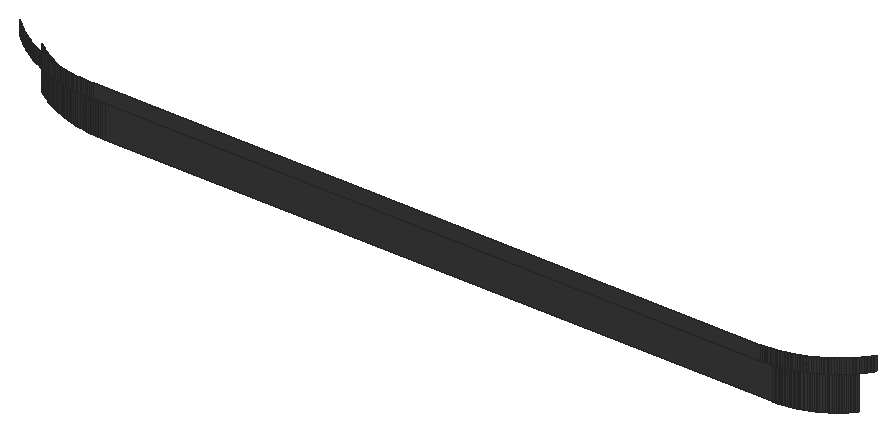
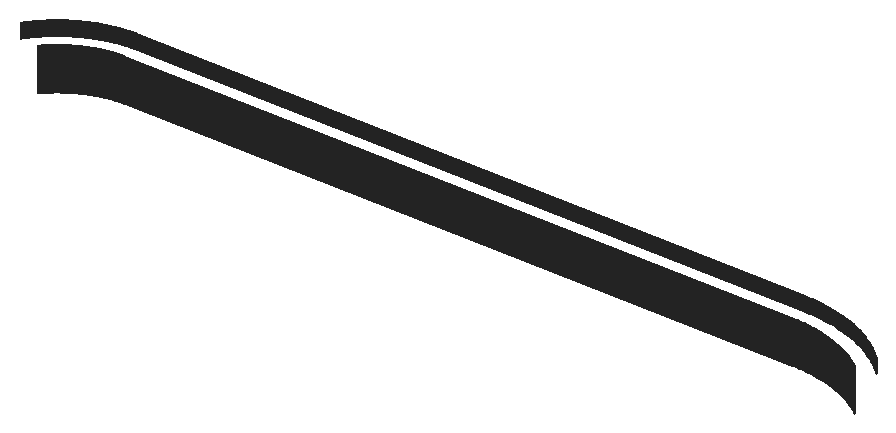
# SketchUp Ruby script. Lengths in inches.
U = 1.inch
M = Sketchup.active_model
def pt(a) = Geom::Point3d.new(a.map { |v| v * U })
def face(e, loops, mat)
  f = e.add_face(loops[0].map { |a| pt(a) })
  loops[1..].each { |l| e.add_face(l.map { |a| pt(a) }).erase! }
  f.material = f.back_material = mat if mat
  f
end
# faces: each face lists its corners as indices into pts; further lists are holes
def faces(e, pts, list, mat = nil) = list.each { |f| face(e, (f[0].is_a?(Array) ? f : [f]).map { |l| l.map { |i| pts[i] } }, mat) }
# xy, xz, yz: faces in a plane at the given z, y or x. An outline is a flat list of corners, or four numbers for a rectangle; further outlines are holes
def ring(l) = l.size == 4 ? [[l[0], l[1]], [l[2], l[1]], [l[2], l[3]], [l[0], l[3]]] : l.each_slice(2).to_a
def flat(e, list, mat, &to3) = list.each { |f| face(e, (f[0].is_a?(Array) ? f : [f]).map { |l| ring(l).map { |u, v| to3.(u, v) } }, mat) }
def xy(e, z, list, mat = nil) = flat(e, list, mat) { |x, y| [x, y, z] }
def xz(e, y, list, mat = nil) = flat(e, list, mat) { |x, z| [x, y, z] }
def yz(e, x, list, mat = nil) = flat(e, list, mat) { |y, z| [x, y, z] }
def lines(e, pts, list) = list.each { |a, b| e.add_line(pt(pts[a]), pt(pts[b])) }
# prism: a flat outline (further loops are holes) pulled along v
def prism(e, loops, v, mat = nil)
  f = face(e, loops, mat); d = Geom::Vector3d.new(v.map { |x| x * U })
  f.pushpull(f.normal.samedirection?(d) ? d.length : -d.length)
end
def box(e, o, s, mat = nil) = prism(e, [[o, [o[0] + s[0], o[1], o[2]], [o[0] + s[0], o[1] + s[1], o[2]], [o[0], o[1] + s[1], o[2]]]], [0, 0, s[2]], mat)
def at(x, y, z, deg = 0) = Geom::Transformation.translation(pt([x, y, z])) * Geom::Transformation.rotation(ORIGIN, Z_AXIS, deg.degrees)
def axes(o, x, y, z) = Geom::Transformation.new([*x, 0, *y, 0, *z, 0, *pt(o).to_a, 1])
def part(name) = M.definitions.add(name)
# library, detail: a bought-in or finely detailed component or shape, given as its bounding box
def library(name, o, s) = part(name).tap { |d| box(d.entities, o, s) }
def detail(e, o, s) = box(e.add_group.entities, o, s)
def put(e, d, t, mat = nil) = e.add_instance(d, t).tap { |i| i.material = mat if mat }
def group(e, t, mat = nil) = e.add_group.tap { |g| g.transformation = t; g.material = mat if mat }.entities
root = M.entities
M.materials.add("1496 AP 8293 CARBON COPY").color = [58, 58, 58]
xz(root,64,[[43.57,270,44,273],[44,270,185,273],[185,270,185.27,273]],"1496 AP 8293 CARBON COPY")
xz(root,67,[[43.61,261,44,270],[44,261,185,270],[185,261,185.24,270]],"1496 AP 8293 CARBON COPY")
xz(root,67.01,[[185.47,261,185.71,270]],"1496 AP 8293 CARBON COPY")
p = [[42.43,67.04,261],[42.43,67.04,270],[42.04,67.0625,270],[42.04,67.0625,261],[42.82,67.02,261],[42.82,67.02,270],
  [43.21,67.01,261],[43.21,67.01,270],[43.61,67,261],[43.61,67,270],[185.47,67.01,261],[185.47,67.01,270],
  [185.24,67,270],[185.24,67,261],[185.94,67.02,261],[185.94,67.02,270],[185.71,67.01,270],[185.71,67.01,261],
  [186.18,67.04,261],[186.18,67.04,270],[186.41,67.06,261],[186.41,67.06,270],[41.25,67.125,261],[41.25,67.125,270],
  [40.86,67.16,270],[40.86,67.16,261],[41.65,67.09,261],[41.65,67.09,270],[186.65,67.08,261],[186.65,67.08,270],
  [186.88,67.1,261],[186.88,67.1,270],[187.12,67.125,261],[187.12,67.125,270],[187.35,67.15,261],[187.35,67.15,270],
  [40.47,67.21,261],[40.47,67.21,270],[40.08,67.26,270],[40.08,67.26,261],[187.58,67.1875,261],[187.58,67.1875,270],
  [187.82,67.22,261],[187.82,67.22,270],[188.05,67.26,261],[188.05,67.26,270],[39.7,67.31,261],[39.7,67.31,270],
  [39.31,67.37,270],[39.31,67.37,261],[188.28,67.3,261],[188.28,67.3,270],[188.51,67.35,261],[188.51,67.35,270],
  [188.74,67.39,261],[188.74,67.39,270],[38.92,67.43,261],[38.92,67.43,270],[38.53,67.5,270],[38.53,67.5,261],
  [188.97,67.44,261],[188.97,67.44,270],[189.2,67.5,261],[189.2,67.5,270],[38.15,67.58,270],[38.15,67.58,261],
  [189.43,67.55,261],[189.43,67.55,270],[37.76,67.66,270],[37.76,67.66,261],[189.66,67.61,261],[189.66,67.61,270],
  [189.89,67.68,261],[189.89,67.68,270],[37.38,67.74,261],[37.38,67.74,270],[37,67.83,270],[37,67.83,261],
  [190.11,67.74,261],[190.11,67.74,270],[190.34,67.81,261],[190.34,67.81,270],[36.62,67.92,270],[36.62,67.92,261],
  [190.5625,67.88,261],[190.5625,67.88,270],[36.24,68.02,270],[36.24,68.02,261],[190.79,67.96,261],[190.79,67.96,270],
  [35.86,68.125,270],[35.86,68.125,261],[191.01,68.03,261],[191.01,68.03,270],[191.23,68.11,261],[191.23,68.11,270],
  [35.48,68.24,270],[35.48,68.24,261],[191.45,68.2,261],[191.45,68.2,270],[35.1,68.35,270],[35.1,68.35,261],
  [191.67,68.28,261],[191.67,68.28,270],[34.73,68.47,270],[34.73,68.47,261],[191.89,68.37,261],[191.89,68.37,270],
  [192.11,68.46,261],[192.11,68.46,270],[34.36,68.59,270],[34.36,68.59,261],[192.32,68.56,261],[192.32,68.56,270],
  [33.99,68.72,270],[33.99,68.72,261],[192.54,68.65,261],[192.54,68.65,270],[33.62,68.85,270],[33.62,68.85,261],
  [192.75,68.75,261],[192.75,68.75,270],[192.96,68.86,261],[192.96,68.86,270],[33.25,68.99,270],[33.25,68.99,261],
  [193.17,68.96,261],[193.17,68.96,270],[32.88,69.14,270],[32.88,69.14,261],[193.38,69.07,261],[193.38,69.07,270],
  [32.52,69.28,270],[32.52,69.28,261],[193.59,69.18,261],[193.59,69.18,270],[193.8,69.3,261],[193.8,69.3,270],
  [32.16,69.4375,270],[32.16,69.4375,261],[194,69.41,261],[194,69.41,270],[31.8,69.59,270],[31.8,69.59,261],
  [194.2,69.53,261],[194.2,69.53,270],[194.4,69.65,261],[194.4,69.65,270],[31.44,69.76,270],[31.44,69.76,261],
  [194.61,69.78,261],[194.61,69.78,270],[31.08,69.92,270],[31.08,69.92,261],[194.8,69.9,261],[194.8,69.9,270],
  [30.73,70.09,270],[30.73,70.09,261],[195,70.03,261],[195,70.03,270],[195.2,70.17,261],[195.2,70.17,270],
  [30.38,70.27,270],[30.38,70.27,261],[195.39,70.3,261],[195.39,70.3,270],[30.03,70.45,270],[30.03,70.45,261],
  [195.58,70.4375,261],[195.58,70.4375,270],[195.77,70.58,261],[195.77,70.58,270],[29.69,70.64,270],[29.69,70.64,261],
  [29.34,70.83,270],[29.34,70.83,261],[195.96,70.72,261],[195.96,70.72,270],[196.14,70.86,261],[196.14,70.86,270],
  [29,71.02,270],[29,71.02,261],[196.33,71.01,261],[196.33,71.01,270],[28.66,71.22,270],[28.66,71.22,261],
  [196.51,71.16,261],[196.51,71.16,270],[28.33,71.42,270],[28.33,71.42,261],[196.69,71.3125,261],[196.69,71.3125,270],
  [196.87,71.47,261],[196.87,71.47,270],[27.99,71.63,270],[27.99,71.63,261],[197.04,71.625,261],[197.04,71.625,270],
  [27.66,71.84,270],[27.66,71.84,261],[197.22,71.78,261],[197.22,71.78,270],[27.33,72.06,270],[27.33,72.06,261],
  [197.39,71.94,261],[197.39,71.94,270],[197.56,72.11,261],[197.56,72.11,270],[27.01,72.28,270],[27.01,72.28,261],
  [197.73,72.27,261],[197.73,72.27,270],[26.6875,72.5,270],[26.6875,72.5,261],[197.89,72.44,261],[197.89,72.44,270],
  [198.06,72.61,261],[198.06,72.61,270],[26.37,72.73,270],[26.37,72.73,261],[198.22,72.78,261],[198.22,72.78,270],
  [26.05,72.96,270],[26.05,72.96,261],[198.375,72.96,261],[198.375,72.96,270],[25.74,73.2,270],[25.74,73.2,261],
  [198.53,73.13,261],[198.53,73.13,270],[41.84,64.07,270],[42.27,64.05,270],[42.27,64.05,273],[41.84,64.07,273],
  [42.7,64.03,270],[42.7,64.03,273],[43.14,64.01,270],[43.14,64.01,273],[43.57,64,270],[43.57,64,273],
  [185.27,64,270],[185.55,64.01,270],[185.55,64.01,273],[185.27,64,273],[185.82,64.02,270],[185.82,64.02,273],
  [186.1,64.03,270],[186.1,64.03,273],[186.375,64.04,270],[186.375,64.04,273],[186.65,64.06,270],[186.65,64.06,273],
  [40.55,64.18,270],[40.98,64.14,270],[40.98,64.14,273],[40.55,64.18,273],[41.41,64.1,270],[41.41,64.1,273],
  [186.92,64.09,270],[186.92,64.09,273],[187.2,64.12,270],[187.2,64.12,273],[187.47,64.15,270],[187.47,64.15,273],
  [187.74,64.18,270],[187.74,64.18,273],[39.69,64.28,270],[40.12,64.23,270],[40.12,64.23,273],[39.69,64.28,273],
  [188.01,64.22,270],[188.01,64.22,273],[188.29,64.26,270],[188.29,64.26,273],[38.84,64.41,270],[39.26,64.34,270],
  [39.26,64.34,273],[38.84,64.41,273],[188.56,64.3,270],[188.56,64.3,273],[188.83,64.35,270],[188.83,64.35,273],
  [38.41,64.48,270],[38.41,64.48,273],[189.1,64.4,270],[189.1,64.4,273],[189.37,64.46,270],[189.37,64.46,273],
  [37.99,64.55,270],[37.99,64.55,273],[189.63,64.52,270],[189.63,64.52,273],[189.9,64.58,270],[189.9,64.58,273],
  [37.14,64.72,270],[37.5625,64.63,270],[37.5625,64.63,273],[37.14,64.72,273],[190.17,64.65,270],[190.17,64.65,273],
  [190.44,64.72,270],[190.44,64.72,273],[36.72,64.8125,270],[36.72,64.8125,273],[190.7,64.79,270],[190.7,64.79,273],
  [36.3,64.91,270],[36.3,64.91,273],[190.96,64.86,270],[190.96,64.86,273],[35.875,65.02,270],[35.875,65.02,273],
  [191.23,64.94,270],[191.23,64.94,273],[191.49,65.03,270],[191.49,65.03,273],[35.46,65.125,270],[35.46,65.125,273],
  [191.75,65.11,270],[191.75,65.11,273],[35.04,65.24,270],[35.04,65.24,273],[192.01,65.2,270],[192.01,65.2,273],
  [34.63,65.36,270],[34.63,65.36,273],[192.27,65.3,270],[192.27,65.3,273],[192.53,65.39,270],[192.53,65.39,273],
  [34.21,65.48,270],[34.21,65.48,273],[192.78,65.49,270],[192.78,65.49,273],[33.8,65.62,270],[33.8,65.62,273],
  [193.04,65.6,270],[193.04,65.6,273],[33.39,65.75,270],[33.39,65.75,273],[193.29,65.71,270],[193.29,65.71,273],
  [193.54,65.82,270],[193.54,65.82,273],[32.98,65.89,270],[32.98,65.89,273],[193.79,65.93,270],[193.79,65.93,273],
  [32.58,66.04,270],[32.58,66.04,273],[194.04,66.05,270],[194.04,66.05,273],[32.17,66.19,270],[32.17,66.19,273],
  [194.29,66.17,270],[194.29,66.17,273],[31.77,66.35,270],[31.77,66.35,273],[194.53,66.29,270],[194.53,66.29,273],
  [31.37,66.51,270],[31.37,66.51,273],[194.78,66.42,270],[194.78,66.42,273],[195.02,66.54,270],[195.02,66.54,273],
  [30.97,66.68,270],[30.97,66.68,273],[195.26,66.68,270],[195.26,66.68,273],[30.58,66.85,270],[30.58,66.85,273],
  [195.5,66.8125,270],[195.5,66.8125,273],[195.74,66.95,270],[195.74,66.95,273],[30.18,67.03,270],[30.18,67.03,273],
  [29.79,67.21,270],[29.79,67.21,273],[195.97,67.09,270],[195.97,67.09,273],[196.21,67.24,270],[196.21,67.24,273],
  [29.4,67.4,270],[29.4,67.4,273],[196.4375,67.39,270],[196.4375,67.39,273],[29.02,67.6,270],[29.02,67.6,273],
  [196.67,67.54,270],[196.67,67.54,273],[196.89,67.69,270],[196.89,67.69,273],[28.63,67.8,270],[28.63,67.8,273],
  [197.12,67.85,270],[197.12,67.85,273],[28.25,68,270],[28.25,68,273],[197.34,68.01,270],[197.34,68.01,273],
  [27.875,68.21,270],[27.875,68.21,273],[197.56,68.17,270],[197.56,68.17,273],[27.5,68.42,270],[27.5,68.42,273],
  [197.78,68.34,270],[197.78,68.34,273],[198,68.51,270],[198,68.51,273],[27.13,68.64,270],[27.13,68.64,273],
  [198.22,68.68,270],[198.22,68.68,273],[26.76,68.86,270],[26.76,68.86,273],[198.43,68.85,270],[198.43,68.85,273],
  [26.39,69.09,270],[26.39,69.09,273],[198.64,69.03,270],[198.64,69.03,273],[198.85,69.21,270],[198.85,69.21,273],
  [26.03,69.32,270],[26.03,69.32,273],[199.05,69.39,270],[199.05,69.39,273],[25.67,69.5625,270],[25.67,69.5625,273],
  [199.25,69.58,270],[199.25,69.58,273],[25.31,69.8,270],[25.31,69.8,273],[199.46,69.77,270],[199.46,69.77,273],
  [24.95,70.05,270],[24.95,70.05,273],[199.65,69.96,270],[199.65,69.96,273],[199.85,70.15,270],[199.85,70.15,273],
  [24.6,70.3,270],[24.6,70.3,273],[200.04,70.35,270],[200.04,70.35,273],[24.26,70.56,270],[24.26,70.56,273],
  [200.23,70.54,270],[200.23,70.54,273],[200.42,70.75,270],[200.42,70.75,273],[23.91,70.82,270],[23.91,70.82,273],
  [200.61,70.95,270],[200.61,70.95,273],[23.57,71.08,270],[23.57,71.08,273],[200.79,71.15,270],[200.79,71.15,273],
  [23.23,71.35,270],[23.23,71.35,273],[200.97,71.36,270],[200.97,71.36,273],[22.9,71.63,270],[22.9,71.63,273],
  [201.15,71.57,270],[201.15,71.57,273],[22.57,71.91,270],[22.57,71.91,273],[201.32,71.78,270],[201.32,71.78,273],
  [201.49,72,270],[201.49,72,273],[22.24,72.1875,270],[22.24,72.1875,273],[201.66,72.22,270],[201.66,72.22,273],
  [21.92,72.48,270],[21.92,72.48,273],[201.83,72.44,270],[201.83,72.44,273],[201.99,72.66,270],[201.99,72.66,273],
  [21.6,72.77,270],[21.6,72.77,273],[202.15,72.88,270],[202.15,72.88,273],[21.28,73.0625,270],[21.28,73.0625,273],
  [202.31,73.11,270],[202.31,73.11,273]]
faces(root,p,[[0,1,2,3],[4,5,1,0],[6,7,5,4],[8,9,7,6],[10,11,12,13],[14,15,16,17],[18,19,15,14],[20,21,19,18],
  [22,23,24,25],[26,27,23,22],[3,2,27,26],[28,29,21,20],[30,31,29,28],[32,33,31,30],[34,35,33,32],[36,37,38,39],
  [25,24,37,36],[40,41,35,34],[42,43,41,40],[44,45,43,42],[46,47,48,49],[39,38,47,46],[50,51,45,44],[52,53,51,50],
  [54,55,53,52],[56,57,58,59],[49,48,57,56],[60,61,55,54],[62,63,61,60],[59,58,64,65],[66,67,63,62],[65,64,68,69],
  [70,71,67,66],[72,73,71,70],[74,75,76,77],[69,68,75,74],[78,79,73,72],[80,81,79,78],[77,76,82,83],[84,85,81,80],
  [83,82,86,87],[88,89,85,84],[87,86,90,91],[92,93,89,88],[94,95,93,92],[91,90,96,97],[98,99,95,94],[97,96,100,101],
  [102,103,99,98],[101,100,104,105],[106,107,103,102],[108,109,107,106],[105,104,110,111],[112,113,109,108],[111,110,114,115],[116,117,113,112],
  [115,114,118,119],[120,121,117,116],[122,123,121,120],[119,118,124,125],[126,127,123,122],[125,124,128,129],[130,131,127,126],[129,128,132,133],
  [134,135,131,130],[136,137,135,134],[133,132,138,139],[140,141,137,136],[139,138,142,143],[144,145,141,140],[146,147,145,144],[143,142,148,149],
  [150,151,147,146],[149,148,152,153],[154,155,151,150],[153,152,156,157],[158,159,155,154],[160,161,159,158],[157,156,162,163],[164,165,161,160],
  [163,162,166,167],[168,169,165,164],[170,171,169,168],[167,166,172,173],[173,172,174,175],[176,177,171,170],[178,179,177,176],[175,174,180,181],
  [182,183,179,178],[181,180,184,185],[186,187,183,182],[185,184,188,189],[190,191,187,186],[192,193,191,190],[189,188,194,195],[196,197,193,192],
  [195,194,198,199],[200,201,197,196],[199,198,202,203],[204,205,201,200],[206,207,205,204],[203,202,208,209],[210,211,207,206],[209,208,212,213],
  [214,215,211,210],[216,217,215,214],[213,212,218,219],[220,221,217,216],[219,218,222,223],[224,225,221,220],[223,222,226,227],[228,229,225,224],
  [230,231,232,233],[231,234,235,232],[234,236,237,235],[236,238,239,237],[240,241,242,243],[241,244,245,242],[244,246,247,245],[246,248,249,247],
  [248,250,251,249],[252,253,254,255],[253,256,257,254],[256,230,233,257],[250,258,259,251],[258,260,261,259],[260,262,263,261],[262,264,265,263],
  [266,267,268,269],[267,252,255,268],[264,270,271,265],[270,272,273,271],[274,275,276,277],[275,266,269,276],[272,278,279,273],[278,280,281,279],
  [282,274,277,283],[280,284,285,281],[284,286,287,285],[288,282,283,289],[286,290,291,287],[290,292,293,291],[294,295,296,297],[295,288,289,296],
  [292,298,299,293],[298,300,301,299],[302,294,297,303],[300,304,305,301],[306,302,303,307],[304,308,309,305],[310,306,307,311],[308,312,313,309],
  [312,314,315,313],[316,310,311,317],[314,318,319,315],[320,316,317,321],[318,322,323,319],[324,320,321,325],[322,326,327,323],[326,328,329,327],
  [330,324,325,331],[328,332,333,329],[334,330,331,335],[332,336,337,333],[338,334,335,339],[336,340,341,337],[340,342,343,341],[344,338,339,345],
  [342,346,347,343],[348,344,345,349],[346,350,351,347],[352,348,349,353],[350,354,355,351],[356,352,353,357],[354,358,359,355],[360,356,357,361],
  [358,362,363,359],[362,364,365,363],[366,360,361,367],[364,368,369,365],[370,366,367,371],[368,372,373,369],[372,374,375,373],[376,370,371,377],
  [378,376,377,379],[374,380,381,375],[380,382,383,381],[384,378,379,385],[382,386,387,383],[388,384,385,389],[386,390,391,387],[390,392,393,391],
  [394,388,389,395],[392,396,397,393],[398,394,395,399],[396,400,401,397],[402,398,399,403],[400,404,405,401],[406,402,403,407],[404,408,409,405],
  [408,410,411,409],[412,406,407,413],[410,414,415,411],[416,412,413,417],[414,418,419,415],[420,416,417,421],[418,422,423,419],[422,424,425,423],
  [426,420,421,427],[424,428,429,425],[430,426,427,431],[428,432,433,429],[434,430,431,435],[432,436,437,433],[438,434,435,439],[436,440,441,437],
  [440,442,443,441],[444,438,439,445],[442,446,447,443],[448,444,445,449],[446,450,451,447],[450,452,453,451],[454,448,449,455],[452,456,457,453],
  [458,454,455,459],[456,460,461,457],[462,458,459,463],[460,464,465,461],[466,462,463,467],[464,468,469,465],[470,466,467,471],[468,472,473,469],
  [472,474,475,473],[476,470,471,477],[474,478,479,475],[480,476,477,481],[478,482,483,479],[482,484,485,483],[486,480,481,487],[484,488,489,485],
  [490,486,487,491],[488,492,493,489]],"1496 AP 8293 CARBON COPY")
